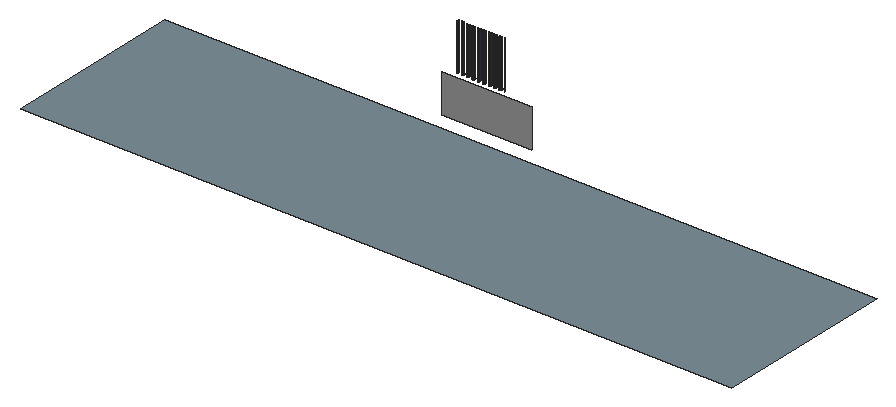
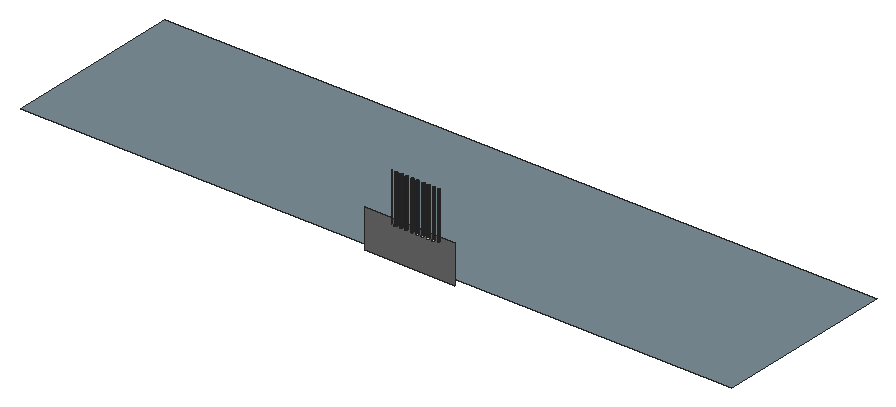
# SketchUp Ruby script. Lengths in inches.
U = 1.inch
M = Sketchup.active_model
def pt(a) = Geom::Point3d.new(a.map { |v| v * U })
def face(e, loops, mat)
  f = e.add_face(loops[0].map { |a| pt(a) })
  loops[1..].each { |l| e.add_face(l.map { |a| pt(a) }).erase! }
  f.material = f.back_material = mat if mat
  f
end
# faces: each face lists its corners as indices into pts; further lists are holes
def faces(e, pts, list, mat = nil) = list.each { |f| face(e, (f[0].is_a?(Array) ? f : [f]).map { |l| l.map { |i| pts[i] } }, mat) }
# xy, xz, yz: faces in a plane at the given z, y or x. An outline is a flat list of corners, or four numbers for a rectangle; further outlines are holes
def ring(l) = l.size == 4 ? [[l[0], l[1]], [l[2], l[1]], [l[2], l[3]], [l[0], l[3]]] : l.each_slice(2).to_a
def flat(e, list, mat, &to3) = list.each { |f| face(e, (f[0].is_a?(Array) ? f : [f]).map { |l| ring(l).map { |u, v| to3.(u, v) } }, mat) }
def xy(e, z, list, mat = nil) = flat(e, list, mat) { |x, y| [x, y, z] }
def xz(e, y, list, mat = nil) = flat(e, list, mat) { |x, z| [x, y, z] }
def yz(e, x, list, mat = nil) = flat(e, list, mat) { |y, z| [x, y, z] }
def lines(e, pts, list) = list.each { |a, b| e.add_line(pt(pts[a]), pt(pts[b])) }
# prism: a flat outline (further loops are holes) pulled along v
def prism(e, loops, v, mat = nil)
  f = face(e, loops, mat); d = Geom::Vector3d.new(v.map { |x| x * U })
  f.pushpull(f.normal.samedirection?(d) ? d.length : -d.length)
end
def box(e, o, s, mat = nil) = prism(e, [[o, [o[0] + s[0], o[1], o[2]], [o[0] + s[0], o[1] + s[1], o[2]], [o[0], o[1] + s[1], o[2]]]], [0, 0, s[2]], mat)
def at(x, y, z, deg = 0) = Geom::Transformation.translation(pt([x, y, z])) * Geom::Transformation.rotation(ORIGIN, Z_AXIS, deg.degrees)
def axes(o, x, y, z) = Geom::Transformation.new([*x, 0, *y, 0, *z, 0, *pt(o).to_a, 1])
def part(name) = M.definitions.add(name)
# library, detail: a bought-in or finely detailed component or shape, given as its bounding box
def library(name, o, s) = part(name).tap { |d| box(d.entities, o, s) }
def detail(e, o, s) = box(e.add_group.entities, o, s)
def put(e, d, t, mat = nil) = e.add_instance(d, t).tap { |i| i.material = mat if mat }
def group(e, t, mat = nil) = e.add_group.tap { |g| g.transformation = t; g.material = mat if mat }.entities
root = M.entities
M.materials.add("[Color M04]").color = [142, 142, 142]
M.materials.add("[Formica Laminate Dark]").color = [50, 53, 60]
M.materials.add("[Square Glass Tile 01]").color = [123, 142, 151]
xy(root,0,[[0,0,377.8125,96.24]],"[Square Glass Tile 01]")
xy(root,22.1875,[[149.83,106,149.65,106.02,149.49,106.09,149.35,106.2,149.24,106.34,149.17,106.51,149.15,106.6875,149.17,106.87,149.24,107.03,149.35,107.17,149.49,107.28,149.65,107.35,149.83,107.375,150.01,107.35,150.18,107.28,150.32,107.17,150.43,107.03,150.5,106.87,150.52,106.6875,150.5,106.51,150.43,106.34,150.32,106.2,150.18,106.09,150.01,106.02],[152.71,106,152.53,106.02,152.36,106.09,152.22,106.2,152.11,106.34,152.04,106.51,152.02,106.6875,152.04,106.87,152.11,107.03,152.22,107.17,152.36,107.28,152.53,107.35,152.71,107.375,152.89,107.35,153.05,107.28,153.19,107.17,153.3,107.03,153.37,106.87,153.4,106.6875,153.37,106.51,153.3,106.34,153.19,106.2,153.05,106.09,152.89,106.02],[155.58,106,155.4,106.02,155.24,106.09,155.1,106.2,154.99,106.34,154.92,106.51,154.9,106.6875,154.92,106.87,154.99,107.03,155.1,107.17,155.24,107.28,155.4,107.35,155.58,107.375,155.76,107.35,155.93,107.28,156.07,107.17,156.18,107.03,156.25,106.87,156.27,106.6875,156.25,106.51,156.18,106.34,156.07,106.2,155.93,106.09,155.76,106.02],[158.46,106,158.28,106.02,158.11,106.09,157.97,106.2,157.86,106.34,157.79,106.51,157.77,106.6875,157.79,106.87,157.86,107.03,157.97,107.17,158.11,107.28,158.28,107.35,158.46,107.375,158.64,107.35,158.8,107.28,158.94,107.17,159.05,107.03,159.12,106.87,159.15,106.6875,159.12,106.51,159.05,106.34,158.94,106.2,158.8,106.09,158.64,106.02],[161.33,106,161.15,106.02,160.99,106.09,160.85,106.2,160.74,106.34,160.67,106.51,160.65,106.6875,160.67,106.87,160.74,107.03,160.85,107.17,160.99,107.28,161.15,107.35,161.33,107.375,161.51,107.35,161.68,107.28,161.82,107.17,161.93,107.03,162,106.87,162.02,106.6875,162,106.51,161.93,106.34,161.82,106.2,161.68,106.09,161.51,106.02],
  [164.21,106,164.03,106.02,163.86,106.09,163.72,106.2,163.61,106.34,163.54,106.51,163.52,106.6875,163.54,106.87,163.61,107.03,163.72,107.17,163.86,107.28,164.03,107.35,164.21,107.375,164.39,107.35,164.55,107.28,164.69,107.17,164.8,107.03,164.87,106.87,164.9,106.6875,164.87,106.51,164.8,106.34,164.69,106.2,164.55,106.09,164.39,106.02],[167.08,106,166.9,106.02,166.74,106.09,166.6,106.2,166.49,106.34,166.42,106.51,166.4,106.6875,166.42,106.87,166.49,107.03,166.6,107.17,166.74,107.28,166.9,107.35,167.08,107.375,167.26,107.35,167.43,107.28,167.57,107.17,167.68,107.03,167.75,106.87,167.77,106.6875,167.75,106.51,167.68,106.34,167.57,106.2,167.43,106.09,167.26,106.02],[169.96,106,169.78,106.02,169.61,106.09,169.47,106.2,169.36,106.34,169.29,106.51,169.27,106.6875,169.29,106.87,169.36,107.03,169.47,107.17,169.61,107.28,169.78,107.35,169.96,107.375,170.14,107.35,170.3,107.28,170.44,107.17,170.55,107.03,170.62,106.87,170.65,106.6875,170.62,106.51,170.55,106.34,170.44,106.2,170.3,106.09,170.14,106.02]])
xz(root,102.91,[[141.86,1.75,189.5,22.1875]],"[Color M04]")
p = [[147.14,106.02,22.1875],[147.3,106.09,22.1875],[147.3,106.09,47.21],[147.14,106.02,47.21],[149.49,106.09,22.1875],[149.65,106.02,22.1875],
  [149.65,106.02,47.21],[149.49,106.09,47.21],[149.83,106,22.1875],[149.83,106,47.21],[150.01,106.02,22.1875],[150.01,106.02,47.21],
  [150.18,106.09,22.1875],[150.18,106.09,47.21],[152.36,106.09,22.1875],[152.53,106.02,22.1875],[152.53,106.02,47.21],[152.36,106.09,47.21],
  [152.71,106,22.1875],[152.71,106,47.21],[152.89,106.02,22.1875],[152.89,106.02,47.21],[153.05,106.09,22.1875],[153.05,106.09,47.21],
  [155.24,106.09,22.1875],[155.4,106.02,22.1875],[155.4,106.02,47.21],[155.24,106.09,47.21],[155.58,106,22.1875],[155.58,106,47.21],
  [155.76,106.02,22.1875],[155.76,106.02,47.21],[155.93,106.09,22.1875],[155.93,106.09,47.21],[158.11,106.09,22.1875],[158.28,106.02,22.1875],
  [158.28,106.02,47.21],[158.11,106.09,47.21],[158.46,106,22.1875],[158.46,106,47.21],[158.64,106.02,22.1875],[158.64,106.02,47.21],
  [158.8,106.09,22.1875],[158.8,106.09,47.21],[160.99,106.09,22.1875],[161.15,106.02,22.1875],[161.15,106.02,47.21],[160.99,106.09,47.21],
  [161.33,106,22.1875],[161.33,106,47.21],[161.51,106.02,22.1875],[161.51,106.02,47.21],[161.68,106.09,22.1875],[161.68,106.09,47.21],
  [163.86,106.09,22.1875],[164.03,106.02,22.1875],[164.03,106.02,47.21],[163.86,106.09,47.21],[164.21,106,22.1875],[164.21,106,47.21],
  [164.39,106.02,22.1875],[164.39,106.02,47.21],[164.55,106.09,22.1875],[164.55,106.09,47.21],[166.74,106.09,22.1875],[166.9,106.02,22.1875],
  [166.9,106.02,47.21],[166.74,106.09,47.21],[167.08,106,22.1875],[167.08,106,47.21],[167.26,106.02,22.1875],[167.26,106.02,47.21],
  [167.43,106.09,22.1875],[167.43,106.09,47.21],[169.61,106.09,22.1875],[169.78,106.02,22.1875],[169.78,106.02,47.21],[169.61,106.09,47.21],
  [169.96,106,22.1875],[169.96,106,47.21],[170.14,106.02,22.1875],[170.14,106.02,47.21],[170.3,106.09,22.1875],[170.3,106.09,47.21],
  [172.49,106.09,22.1875],[172.65,106.02,22.1875],[172.65,106.02,47.21],[172.49,106.09,47.21],[147.44,106.2,22.1875],[147.44,106.2,47.21],
  [149.35,106.2,22.1875],[149.35,106.2,47.21],[150.32,106.2,22.1875],[150.32,106.2,47.21],[152.22,106.2,22.1875],[152.22,106.2,47.21],
  [153.19,106.2,22.1875],[153.19,106.2,47.21],[155.1,106.2,22.1875],[155.1,106.2,47.21],[156.07,106.2,22.1875],[156.07,106.2,47.21],
  [157.97,106.2,22.1875],[157.97,106.2,47.21],[158.94,106.2,22.1875],[158.94,106.2,47.21],[160.85,106.2,22.1875],[160.85,106.2,47.21],
  [161.82,106.2,22.1875],[161.82,106.2,47.21],[163.72,106.2,22.1875],[163.72,106.2,47.21],[164.69,106.2,22.1875],[164.69,106.2,47.21],
  [166.6,106.2,22.1875],[166.6,106.2,47.21],[167.57,106.2,22.1875],[167.57,106.2,47.21],[169.47,106.2,22.1875],[169.47,106.2,47.21],
  [170.44,106.2,22.1875],[170.44,106.2,47.21],[172.35,106.2,22.1875],[172.35,106.2,47.21],[147.55,106.34,22.1875],[147.55,106.34,47.21],
  [149.24,106.34,22.1875],[149.24,106.34,47.21],[150.43,106.34,22.1875],[150.43,106.34,47.21],[152.11,106.34,22.1875],[152.11,106.34,47.21],
  [153.3,106.34,22.1875],[153.3,106.34,47.21],[154.99,106.34,22.1875],[154.99,106.34,47.21],[156.18,106.34,22.1875],[156.18,106.34,47.21],
  [157.86,106.34,22.1875],[157.86,106.34,47.21],[159.05,106.34,22.1875],[159.05,106.34,47.21],[160.74,106.34,22.1875],[160.74,106.34,47.21],
  [161.93,106.34,22.1875],[161.93,106.34,47.21],[163.61,106.34,22.1875],[163.61,106.34,47.21],[164.8,106.34,22.1875],[164.8,106.34,47.21],
  [166.49,106.34,22.1875],[166.49,106.34,47.21],[167.68,106.34,22.1875],[167.68,106.34,47.21],[169.36,106.34,22.1875],[169.36,106.34,47.21],
  [170.55,106.34,22.1875],[170.55,106.34,47.21],[172.24,106.34,22.1875],[172.24,106.34,47.21],[147.62,106.51,22.1875],[147.62,106.51,47.21],
  [149.17,106.51,22.1875],[149.17,106.51,47.21],[150.5,106.51,22.1875],[150.5,106.51,47.21],[152.04,106.51,22.1875],[152.04,106.51,47.21],
  [153.37,106.51,22.1875],[153.37,106.51,47.21],[154.92,106.51,22.1875],[154.92,106.51,47.21],[156.25,106.51,22.1875],[156.25,106.51,47.21],
  [157.79,106.51,22.1875],[157.79,106.51,47.21],[159.12,106.51,22.1875],[159.12,106.51,47.21],[160.67,106.51,22.1875],[160.67,106.51,47.21],
  [162,106.51,22.1875],[162,106.51,47.21],[163.54,106.51,22.1875],[163.54,106.51,47.21],[164.87,106.51,22.1875],[164.87,106.51,47.21],
  [166.42,106.51,22.1875],[166.42,106.51,47.21],[167.75,106.51,22.1875],[167.75,106.51,47.21],[169.29,106.51,22.1875],[169.29,106.51,47.21],
  [170.62,106.51,22.1875],[170.62,106.51,47.21],[172.17,106.51,22.1875],[172.17,106.51,47.21],[147.65,106.6875,22.1875],[147.65,106.6875,47.21],
  [149.15,106.6875,22.1875],[149.15,106.6875,47.21],[150.52,106.6875,22.1875],[150.52,106.6875,47.21],[152.02,106.6875,22.1875],[152.02,106.6875,47.21],
  [153.4,106.6875,22.1875],[153.4,106.6875,47.21],[154.9,106.6875,22.1875],[154.9,106.6875,47.21],[156.27,106.6875,22.1875],[156.27,106.6875,47.21],
  [157.77,106.6875,22.1875],[157.77,106.6875,47.21],[159.15,106.6875,22.1875],[159.15,106.6875,47.21],[160.65,106.6875,22.1875],[160.65,106.6875,47.21],
  [162.02,106.6875,22.1875],[162.02,106.6875,47.21],[163.52,106.6875,22.1875],[163.52,106.6875,47.21],[164.9,106.6875,22.1875],[164.9,106.6875,47.21],
  [166.4,106.6875,22.1875],[166.4,106.6875,47.21],[167.77,106.6875,22.1875],[167.77,106.6875,47.21],[169.27,106.6875,22.1875],[169.27,106.6875,47.21],
  [170.65,106.6875,22.1875],[170.65,106.6875,47.21],[172.15,106.6875,22.1875],[172.15,106.6875,47.21],[147.62,106.87,22.1875],[147.62,106.87,47.21],
  [149.17,106.87,22.1875],[149.17,106.87,47.21]]
faces(root,p,[[0,1,2,3],[4,5,6,7],[5,8,9,6],[8,10,11,9],[10,12,13,11],[14,15,16,17],[15,18,19,16],[18,20,21,19],
  [20,22,23,21],[24,25,26,27],[25,28,29,26],[28,30,31,29],[30,32,33,31],[34,35,36,37],[35,38,39,36],[38,40,41,39],
  [40,42,43,41],[44,45,46,47],[45,48,49,46],[48,50,51,49],[50,52,53,51],[54,55,56,57],[55,58,59,56],[58,60,61,59],
  [60,62,63,61],[64,65,66,67],[65,68,69,66],[68,70,71,69],[70,72,73,71],[74,75,76,77],[75,78,79,76],[78,80,81,79],
  [80,82,83,81],[84,85,86,87],[1,88,89,2],[90,4,7,91],[12,92,93,13],[94,14,17,95],[22,96,97,23],[98,24,27,99],
  [32,100,101,33],[102,34,37,103],[42,104,105,43],[106,44,47,107],[52,108,109,53],[110,54,57,111],[62,112,113,63],[114,64,67,115],
  [72,116,117,73],[118,74,77,119],[82,120,121,83],[122,84,87,123],[88,124,125,89],[126,90,91,127],[92,128,129,93],[130,94,95,131],
  [96,132,133,97],[134,98,99,135],[100,136,137,101],[138,102,103,139],[104,140,141,105],[142,106,107,143],[108,144,145,109],[146,110,111,147],
  [112,148,149,113],[150,114,115,151],[116,152,153,117],[154,118,119,155],[120,156,157,121],[158,122,123,159],[124,160,161,125],[162,126,127,163],
  [128,164,165,129],[166,130,131,167],[132,168,169,133],[170,134,135,171],[136,172,173,137],[174,138,139,175],[140,176,177,141],[178,142,143,179],
  [144,180,181,145],[182,146,147,183],[148,184,185,149],[186,150,151,187],[152,188,189,153],[190,154,155,191],[156,192,193,157],[194,158,159,195],
  [160,196,197,161],[198,162,163,199],[164,200,201,165],[202,166,167,203],[168,204,205,169],[206,170,171,207],[172,208,209,173],[210,174,175,211],
  [176,212,213,177],[214,178,179,215],[180,216,217,181],[218,182,183,219],[184,220,221,185],[222,186,187,223],[188,224,225,189],[226,190,191,227],
  [192,228,229,193],[230,194,195,231],[196,232,233,197],[234,198,199,235]],"[Formica Laminate Dark]")
